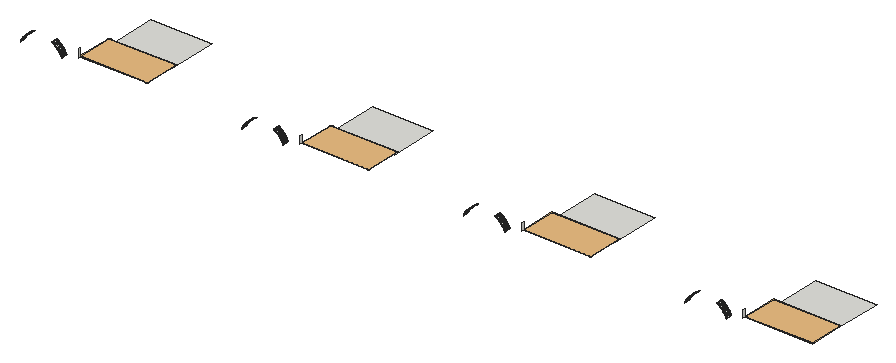
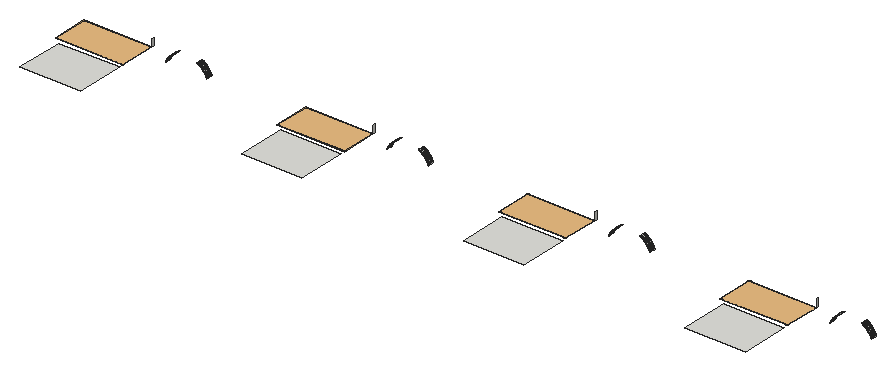
# SketchUp Ruby script. Lengths in inches.
U = 1.inch
M = Sketchup.active_model
def pt(a) = Geom::Point3d.new(a.map { |v| v * U })
def face(e, loops, mat)
  f = e.add_face(loops[0].map { |a| pt(a) })
  loops[1..].each { |l| e.add_face(l.map { |a| pt(a) }).erase! }
  f.material = f.back_material = mat if mat
  f
end
# faces: each face lists its corners as indices into pts; further lists are holes
def faces(e, pts, list, mat = nil) = list.each { |f| face(e, (f[0].is_a?(Array) ? f : [f]).map { |l| l.map { |i| pts[i] } }, mat) }
# xy, xz, yz: faces in a plane at the given z, y or x. An outline is a flat list of corners, or four numbers for a rectangle; further outlines are holes
def ring(l) = l.size == 4 ? [[l[0], l[1]], [l[2], l[1]], [l[2], l[3]], [l[0], l[3]]] : l.each_slice(2).to_a
def flat(e, list, mat, &to3) = list.each { |f| face(e, (f[0].is_a?(Array) ? f : [f]).map { |l| ring(l).map { |u, v| to3.(u, v) } }, mat) }
def xy(e, z, list, mat = nil) = flat(e, list, mat) { |x, y| [x, y, z] }
def xz(e, y, list, mat = nil) = flat(e, list, mat) { |x, z| [x, y, z] }
def yz(e, x, list, mat = nil) = flat(e, list, mat) { |y, z| [x, y, z] }
def lines(e, pts, list) = list.each { |a, b| e.add_line(pt(pts[a]), pt(pts[b])) }
# prism: a flat outline (further loops are holes) pulled along v
def prism(e, loops, v, mat = nil)
  f = face(e, loops, mat); d = Geom::Vector3d.new(v.map { |x| x * U })
  f.pushpull(f.normal.samedirection?(d) ? d.length : -d.length)
end
def box(e, o, s, mat = nil) = prism(e, [[o, [o[0] + s[0], o[1], o[2]], [o[0] + s[0], o[1] + s[1], o[2]], [o[0], o[1] + s[1], o[2]]]], [0, 0, s[2]], mat)
def at(x, y, z, deg = 0) = Geom::Transformation.translation(pt([x, y, z])) * Geom::Transformation.rotation(ORIGIN, Z_AXIS, deg.degrees)
def axes(o, x, y, z) = Geom::Transformation.new([*x, 0, *y, 0, *z, 0, *pt(o).to_a, 1])
def part(name) = M.definitions.add(name)
# library, detail: a bought-in or finely detailed component or shape, given as its bounding box
def library(name, o, s) = part(name).tap { |d| box(d.entities, o, s) }
def detail(e, o, s) = box(e.add_group.entities, o, s)
def put(e, d, t, mat = nil) = e.add_instance(d, t).tap { |i| i.material = mat if mat }
def group(e, t, mat = nil) = e.add_group.tap { |g| g.transformation = t; g.material = mat if mat }.entities
root = M.entities
M.materials.add("[Wood Cherry Original]").color = [152, 86, 42]
c1 = library("Group158\#2",[-67.5,-36,0],[135,72,0.25])
xy(root,249,[[301,301.25,422,398.125],[745,301.25,866,398.125],[1189,301.25,1310,398.125],[1633,301.25,1754,398.125]])
yz(root,294,[[224.6875,256,229.25,271]])
yz(root,738,[[224.6875,256,229.25,271]])
yz(root,1182,[[224.6875,256,229.25,271]])
yz(root,1626,[[224.6875,256,229.25,271]])
p = [[177.72,236.25,243.7],[177.72,224.6875,243.7],[177.48,224.6875,243.13],[177.48,236.25,243.13],[260.65,236.25,243.06],[260.65,224.6875,243.06],
  [260.41,224.6875,243.62],[260.41,236.25,243.62],[621.72,236.25,243.7],[621.72,224.6875,243.7],[621.48,224.6875,243.13],[621.48,236.25,243.13],
  [704.65,236.25,243.06],[704.65,224.6875,243.06],[704.41,224.6875,243.62],[704.41,236.25,243.62],[1065.72,236.25,243.7],[1065.72,224.6875,243.7],
  [1065.48,224.6875,243.13],[1065.48,236.25,243.13],[1148.65,236.25,243.06],[1148.65,224.6875,243.06],[1148.41,224.6875,243.62],[1148.41,236.25,243.62],
  [1509.72,236.25,243.7],[1509.72,224.6875,243.7],[1509.48,224.6875,243.13],[1509.48,236.25,243.13],[1592.65,236.25,243.06],[1592.65,224.6875,243.06],
  [1592.41,224.6875,243.62],[1592.41,236.25,243.62],[260.17,224.6875,244.18],[260.17,236.25,244.18],[704.17,224.6875,244.18],[704.17,236.25,244.18],
  [1148.17,224.6875,244.18],[1148.17,236.25,244.18],[1592.17,224.6875,244.18],[1592.17,236.25,244.18],[177.97,236.25,244.26],[177.97,224.6875,244.26],
  [621.97,236.25,244.26],[621.97,224.6875,244.26],[1065.97,236.25,244.26],[1065.97,224.6875,244.26],[1509.97,236.25,244.26],[1509.97,224.6875,244.26],
  [259.92,224.6875,244.74],[259.92,236.25,244.74],[703.92,224.6875,244.74],[703.92,236.25,244.74],[1147.92,224.6875,244.74],[1147.92,236.25,244.74],
  [1591.92,224.6875,244.74],[1591.92,236.25,244.74],[178.22,236.25,244.83],[178.22,224.6875,244.83],[622.22,236.25,244.83],[622.22,224.6875,244.83],
  [1066.22,236.25,244.83],[1066.22,224.6875,244.83],[1510.22,236.25,244.83],[1510.22,224.6875,244.83],[259.66,224.6875,245.3],[259.66,236.25,245.3],
  [703.66,224.6875,245.3],[703.66,236.25,245.3],[1147.66,224.6875,245.3],[1147.66,236.25,245.3],[1591.66,224.6875,245.3],[1591.66,236.25,245.3],
  [178.48,236.25,245.38],[178.48,224.6875,245.38],[622.48,236.25,245.38],[622.48,224.6875,245.38],[1066.48,236.25,245.38],[1066.48,224.6875,245.38],
  [1510.48,236.25,245.38],[1510.48,224.6875,245.38],[259.39,224.6875,245.85],[259.39,236.25,245.85],[703.39,224.6875,245.85],[703.39,236.25,245.85],
  [1147.39,224.6875,245.85],[1147.39,236.25,245.85],[1591.39,224.6875,245.85],[1591.39,236.25,245.85],[178.75,236.25,245.94],[178.75,224.6875,245.94],
  [622.75,236.25,245.94],[622.75,224.6875,245.94],[1066.75,236.25,245.94],[1066.75,224.6875,245.94],[1510.75,236.25,245.94],[1510.75,224.6875,245.94],
  [259.12,224.6875,246.39],[259.12,236.25,246.39],[703.12,224.6875,246.39],[703.12,236.25,246.39],[1147.12,224.6875,246.39],[1147.12,236.25,246.39],
  [1591.12,224.6875,246.39],[1591.12,236.25,246.39],[179.02,236.25,246.49],[179.02,224.6875,246.49],[623.02,236.25,246.49],[623.02,224.6875,246.49],
  [1067.02,236.25,246.49],[1067.02,224.6875,246.49],[1511.02,236.25,246.49],[1511.02,224.6875,246.49],[258.84,224.6875,246.9375],[258.84,236.25,246.9375],
  [702.84,224.6875,246.9375],[702.84,236.25,246.9375],[1146.84,224.6875,246.9375],[1146.84,236.25,246.9375],[1590.84,224.6875,246.9375],[1590.84,236.25,246.9375],
  [179.31,236.25,247.04],[179.31,224.6875,247.04],[623.31,236.25,247.04],[623.31,224.6875,247.04],[1067.31,236.25,247.04],[1067.31,224.6875,247.04],
  [1511.31,236.25,247.04],[1511.31,224.6875,247.04],[258.55,224.6875,247.48],[258.55,236.25,247.48],[702.55,224.6875,247.48],[702.55,236.25,247.48],
  [1146.55,224.6875,247.48],[1146.55,236.25,247.48],[1590.55,224.6875,247.48],[1590.55,236.25,247.48],[179.6,236.25,247.58],[179.6,224.6875,247.58],
  [623.6,236.25,247.58],[623.6,224.6875,247.58],[1067.6,236.25,247.58],[1067.6,224.6875,247.58],[1511.6,236.25,247.58],[1511.6,224.6875,247.58],
  [258.26,224.6875,248.01],[258.26,236.25,248.01],[702.26,224.6875,248.01],[702.26,236.25,248.01],[1146.26,224.6875,248.01],[1146.26,236.25,248.01],
  [1590.26,224.6875,248.01],[1590.26,236.25,248.01],[179.9,236.25,248.12],[179.9,224.6875,248.12],[623.9,236.25,248.12],[623.9,224.6875,248.12],
  [1067.9,236.25,248.12],[1067.9,224.6875,248.12],[1511.9,236.25,248.12],[1511.9,224.6875,248.12],[257.95,224.6875,248.54],[257.95,236.25,248.54],
  [701.95,224.6875,248.54],[701.95,236.25,248.54],[1145.95,224.6875,248.54],[1145.95,236.25,248.54],[1589.95,224.6875,248.54],[1589.95,236.25,248.54],
  [180.2,236.25,248.66],[180.2,224.6875,248.66],[624.2,236.25,248.66],[624.2,224.6875,248.66],[1068.2,236.25,248.66],[1068.2,224.6875,248.66],
  [1512.2,236.25,248.66],[1512.2,224.6875,248.66],[257.64,224.6875,249.07],[257.64,236.25,249.07],[701.64,224.6875,249.07],[701.64,236.25,249.07],
  [1145.64,224.6875,249.07],[1145.64,236.25,249.07],[1589.64,224.6875,249.07],[1589.64,236.25,249.07],[180.52,236.25,249.19],[180.52,224.6875,249.19],
  [624.52,236.25,249.19],[624.52,224.6875,249.19],[1068.52,236.25,249.19],[1068.52,224.6875,249.19],[1512.52,236.25,249.19],[1512.52,224.6875,249.19],
  [257.33,224.6875,249.59],[257.33,236.25,249.59],[701.33,224.6875,249.59],[701.33,236.25,249.59],[1145.33,224.6875,249.59],[1145.33,236.25,249.59],
  [1589.33,224.6875,249.59],[1589.33,236.25,249.59],[180.84,236.25,249.72],[180.84,224.6875,249.72],[624.84,236.25,249.72],[624.84,224.6875,249.72],
  [1068.84,236.25,249.72],[1068.84,224.6875,249.72],[1512.84,236.25,249.72],[1512.84,224.6875,249.72],[257,224.6875,250.11],[257,236.25,250.11],
  [701,224.6875,250.11],[701,236.25,250.11],[1145,224.6875,250.11],[1145,236.25,250.11],[1589,224.6875,250.11],[1589,236.25,250.11],
  [181.16,236.25,250.24],[181.16,224.6875,250.24],[625.16,236.25,250.24],[625.16,224.6875,250.24],[1069.16,236.25,250.24],[1069.16,224.6875,250.24],
  [1513.16,236.25,250.24],[1513.16,224.6875,250.24],[256.67,224.6875,250.625],[256.67,236.25,250.625],[700.67,224.6875,250.625],[700.67,236.25,250.625],
  [1144.67,224.6875,250.625],[1144.67,236.25,250.625],[1588.67,224.6875,250.625],[1588.67,236.25,250.625],[181.5,236.25,250.76],[181.5,224.6875,250.76],
  [625.5,236.25,250.76],[625.5,224.6875,250.76],[1069.5,236.25,250.76],[1069.5,224.6875,250.76],[1513.5,236.25,250.76],[1513.5,224.6875,250.76],
  [256.33,224.6875,251.13],[256.33,236.25,251.13],[700.33,224.6875,251.13],[700.33,236.25,251.13],[1144.33,224.6875,251.13],[1144.33,236.25,251.13],
  [1588.33,224.6875,251.13],[1588.33,236.25,251.13],[181.84,236.25,251.27],[181.84,224.6875,251.27],[625.84,236.25,251.27],[625.84,224.6875,251.27],
  [1069.84,236.25,251.27],[1069.84,224.6875,251.27],[1513.84,236.25,251.27],[1513.84,224.6875,251.27],[255.99,224.6875,251.64],[255.99,236.25,251.64],
  [699.99,224.6875,251.64],[699.99,236.25,251.64],[1143.99,224.6875,251.64],[1143.99,236.25,251.64],[1587.99,224.6875,251.64],[1587.99,236.25,251.64],
  [182.19,236.25,251.78],[182.19,224.6875,251.78],[626.19,236.25,251.78],[626.19,224.6875,251.78],[1070.19,236.25,251.78],[1070.19,224.6875,251.78],
  [1514.19,236.25,251.78],[1514.19,224.6875,251.78],[255.64,224.6875,252.14],[255.64,236.25,252.14],[699.64,224.6875,252.14],[699.64,236.25,252.14],
  [1143.64,224.6875,252.14],[1143.64,236.25,252.14],[1587.64,224.6875,252.14],[1587.64,236.25,252.14],[182.55,236.25,252.28],[182.55,224.6875,252.28],
  [626.55,236.25,252.28],[626.55,224.6875,252.28],[1070.55,236.25,252.28],[1070.55,224.6875,252.28],[1514.55,236.25,252.28],[1514.55,224.6875,252.28],
  [255.28,224.6875,252.63],[255.28,236.25,252.63],[699.28,224.6875,252.63],[699.28,236.25,252.63],[1143.28,224.6875,252.63],[1143.28,236.25,252.63],
  [1587.28,224.6875,252.63],[1587.28,236.25,252.63],[182.91,236.25,252.78],[182.91,224.6875,252.78],[626.91,236.25,252.78],[626.91,224.6875,252.78],
  [1070.91,236.25,252.78],[1070.91,224.6875,252.78],[1514.91,236.25,252.78],[1514.91,224.6875,252.78],[254.91,224.6875,253.125],[254.91,236.25,253.125],
  [698.91,224.6875,253.125],[698.91,236.25,253.125],[1142.91,224.6875,253.125],[1142.91,236.25,253.125],[1586.91,224.6875,253.125],[1586.91,236.25,253.125],
  [183.28,236.25,253.27],[183.28,224.6875,253.27],[627.28,236.25,253.27],[627.28,224.6875,253.27],[1071.28,236.25,253.27],[1071.28,224.6875,253.27],
  [1515.28,236.25,253.27],[1515.28,224.6875,253.27],[254.54,224.6875,253.61],[254.54,236.25,253.61],[698.54,224.6875,253.61],[698.54,236.25,253.61],
  [1142.54,224.6875,253.61],[1142.54,236.25,253.61],[1586.54,224.6875,253.61],[1586.54,236.25,253.61],[183.65,236.25,253.76],[183.65,224.6875,253.76],
  [627.65,236.25,253.76],[627.65,224.6875,253.76],[1071.65,236.25,253.76],[1071.65,224.6875,253.76],[1515.65,236.25,253.76],[1515.65,224.6875,253.76],
  [254.16,224.6875,254.09],[254.16,236.25,254.09],[698.16,224.6875,254.09],[698.16,236.25,254.09],[1142.16,224.6875,254.09],[1142.16,236.25,254.09],
  [1586.16,224.6875,254.09],[1586.16,236.25,254.09],[184.04,236.25,254.25],[184.04,224.6875,254.25],[628.04,236.25,254.25],[628.04,224.6875,254.25],
  [1072.04,236.25,254.25],[1072.04,224.6875,254.25],[1516.04,236.25,254.25],[1516.04,224.6875,254.25],[253.78,224.6875,254.5625],[253.78,236.25,254.5625],
  [697.78,224.6875,254.5625],[697.78,236.25,254.5625],[1141.78,224.6875,254.5625],[1141.78,236.25,254.5625],[1585.78,224.6875,254.5625],[1585.78,236.25,254.5625],
  [184.43,236.25,254.72],[184.43,224.6875,254.72],[628.43,236.25,254.72],[628.43,224.6875,254.72],[1072.43,236.25,254.72],[1072.43,224.6875,254.72],
  [1516.43,236.25,254.72],[1516.43,224.6875,254.72],[253.39,224.6875,255.03],[253.39,236.25,255.03],[697.39,224.6875,255.03],[697.39,236.25,255.03],
  [1141.39,224.6875,255.03],[1141.39,236.25,255.03],[1585.39,224.6875,255.03],[1585.39,236.25,255.03],[184.82,236.25,255.2],[184.82,224.6875,255.2],
  [628.82,236.25,255.2],[628.82,224.6875,255.2],[1072.82,236.25,255.2],[1072.82,224.6875,255.2],[1516.82,236.25,255.2],[1516.82,224.6875,255.2],
  [252.99,224.6875,255.5],[252.99,236.25,255.5],[696.99,224.6875,255.5],[696.99,236.25,255.5],[1140.99,224.6875,255.5],[1140.99,236.25,255.5],
  [1584.99,224.6875,255.5],[1584.99,236.25,255.5],[185.23,236.25,255.66],[185.23,224.6875,255.66],[629.23,236.25,255.66],[629.23,224.6875,255.66],
  [1073.23,236.25,255.66],[1073.23,224.6875,255.66],[1517.23,236.25,255.66],[1517.23,224.6875,255.66],[252.58,224.6875,255.96],[252.58,236.25,255.96],
  [696.58,224.6875,255.96],[696.58,236.25,255.96],[1140.58,224.6875,255.96],[1140.58,236.25,255.96],[1584.58,224.6875,255.96],[1584.58,236.25,255.96],
  [185.64,236.25,256.125],[185.64,224.6875,256.125],[629.64,236.25,256.125],[629.64,224.6875,256.125],[1073.64,236.25,256.125],[1073.64,224.6875,256.125],
  [1517.64,236.25,256.125],[1517.64,224.6875,256.125],[252.17,224.6875,256.41],[252.17,236.25,256.41],[696.17,224.6875,256.41],[696.17,236.25,256.41],
  [1140.17,224.6875,256.41],[1140.17,236.25,256.41],[1584.17,224.6875,256.41],[1584.17,236.25,256.41],[186.05,236.25,256.58],[186.05,224.6875,256.58],
  [630.05,236.25,256.58],[630.05,224.6875,256.58],[1074.05,236.25,256.58],[1074.05,224.6875,256.58],[1518.05,236.25,256.58],[1518.05,224.6875,256.58],
  [251.76,224.6875,256.86],[251.76,236.25,256.86],[695.76,224.6875,256.86],[695.76,236.25,256.86],[1139.76,224.6875,256.86],[1139.76,236.25,256.86],
  [1583.76,224.6875,256.86],[1583.76,236.25,256.86],[186.47,236.25,257.03],[186.47,224.6875,257.03],[630.47,236.25,257.03],[630.47,224.6875,257.03],
  [1074.47,236.25,257.03],[1074.47,224.6875,257.03],[1518.47,236.25,257.03],[1518.47,224.6875,257.03],[251.34,224.6875,257.3],[251.34,236.25,257.3],
  [695.34,224.6875,257.3],[695.34,236.25,257.3],[1139.34,224.6875,257.3],[1139.34,236.25,257.3],[1583.34,224.6875,257.3],[1583.34,236.25,257.3],
  [186.9,236.25,257.48],[186.9,224.6875,257.48],[630.9,236.25,257.48],[630.9,224.6875,257.48],[1074.9,236.25,257.48],[1074.9,224.6875,257.48],
  [1518.9,236.25,257.48],[1518.9,224.6875,257.48],[250.91,224.6875,257.74],[250.91,236.25,257.74],[694.91,224.6875,257.74],[694.91,236.25,257.74],
  [1138.91,224.6875,257.74],[1138.91,236.25,257.74],[1582.91,224.6875,257.74],[1582.91,236.25,257.74],[187.33,236.25,257.91],[187.33,224.6875,257.91],
  [631.33,236.25,257.91],[631.33,224.6875,257.91],[1075.33,236.25,257.91],[1075.33,224.6875,257.91],[1519.33,236.25,257.91],[1519.33,224.6875,257.91],
  [250.47,224.6875,258.17],[250.47,236.25,258.17],[694.47,224.6875,258.17],[694.47,236.25,258.17],[1138.47,224.6875,258.17],[1138.47,236.25,258.17],
  [1582.47,224.6875,258.17],[1582.47,236.25,258.17],[187.77,236.25,258.35],[187.77,224.6875,258.35],[631.77,236.25,258.35],[631.77,224.6875,258.35],
  [1075.77,236.25,258.35],[1075.77,224.6875,258.35],[1519.77,236.25,258.35],[1519.77,224.6875,258.35],[250.03,224.6875,258.59],[250.03,236.25,258.59],
  [694.03,224.6875,258.59],[694.03,236.25,258.59],[1138.03,224.6875,258.59],[1138.03,236.25,258.59],[1582.03,224.6875,258.59],[1582.03,236.25,258.59],
  [188.22,236.25,258.77],[188.22,224.6875,258.77],[632.22,236.25,258.77],[632.22,224.6875,258.77],[1076.22,236.25,258.77],[1076.22,224.6875,258.77],
  [1520.22,236.25,258.77],[1520.22,224.6875,258.77],[249.59,224.6875,259.01],[249.59,236.25,259.01],[693.59,224.6875,259.01],[693.59,236.25,259.01],
  [1137.59,224.6875,259.01],[1137.59,236.25,259.01],[1581.59,224.6875,259.01],[1581.59,236.25,259.01],[188.67,236.25,259.19],[188.67,224.6875,259.19],
  [632.67,236.25,259.19],[632.67,224.6875,259.19],[1076.67,236.25,259.19],[1076.67,224.6875,259.19],[1520.67,236.25,259.19],[1520.67,224.6875,259.19],
  [249.14,224.6875,259.42],[249.14,236.25,259.42],[693.14,224.6875,259.42],[693.14,236.25,259.42],[1137.14,224.6875,259.42],[1137.14,236.25,259.42],
  [1581.14,224.6875,259.42],[1581.14,236.25,259.42],[189.13,236.25,259.61],[189.13,224.6875,259.61],[633.13,236.25,259.61],[633.13,224.6875,259.61],
  [1077.13,236.25,259.61],[1077.13,224.6875,259.61],[1521.13,236.25,259.61],[1521.13,224.6875,259.61],[248.68,224.6875,259.83],[248.68,236.25,259.83],
  [692.68,224.6875,259.83],[692.68,236.25,259.83],[1136.68,224.6875,259.83],[1136.68,236.25,259.83],[1580.68,224.6875,259.83],[1580.68,236.25,259.83],
  [189.59,236.25,260.02],[189.59,224.6875,260.02],[633.59,236.25,260.02],[633.59,224.6875,260.02],[1077.59,236.25,260.02],[1077.59,224.6875,260.02],
  [1521.59,236.25,260.02],[1521.59,224.6875,260.02],[248.22,224.6875,260.23],[248.22,236.25,260.23],[692.22,224.6875,260.23],[692.22,236.25,260.23],
  [1136.22,224.6875,260.23],[1136.22,236.25,260.23],[1580.22,224.6875,260.23],[1580.22,236.25,260.23],[190.06,236.25,260.42],[190.06,224.6875,260.42],
  [634.06,236.25,260.42],[634.06,224.6875,260.42],[1078.06,236.25,260.42],[1078.06,224.6875,260.42],[1522.06,236.25,260.42],[1522.06,224.6875,260.42],
  [247.75,224.6875,260.625],[247.75,236.25,260.625],[691.75,224.6875,260.625],[691.75,236.25,260.625],[1135.75,224.6875,260.625],[1135.75,236.25,260.625],
  [1579.75,224.6875,260.625],[1579.75,236.25,260.625],[190.53,236.25,260.8125],[190.53,224.6875,260.8125],[634.53,236.25,260.8125],[634.53,224.6875,260.8125],
  [1078.53,236.25,260.8125],[1078.53,224.6875,260.8125],[1522.53,236.25,260.8125],[1522.53,224.6875,260.8125],[247.28,224.6875,261.01],[247.28,236.25,261.01],
  [691.28,224.6875,261.01],[691.28,236.25,261.01],[1135.28,224.6875,261.01],[1135.28,236.25,261.01],[1579.28,224.6875,261.01],[1579.28,236.25,261.01],
  [191.01,236.25,261.2],[191.01,224.6875,261.2],[635.01,236.25,261.2],[635.01,224.6875,261.2],[1079.01,236.25,261.2],[1079.01,224.6875,261.2],
  [1523.01,236.25,261.2],[1523.01,224.6875,261.2],[246.8,224.6875,261.39],[246.8,236.25,261.39],[690.8,224.6875,261.39],[690.8,236.25,261.39],
  [1134.8,224.6875,261.39],[1134.8,236.25,261.39],[1578.8,224.6875,261.39],[1578.8,236.25,261.39],[191.5,236.25,261.58],[191.5,224.6875,261.58],
  [635.5,236.25,261.58],[635.5,224.6875,261.58],[1079.5,236.25,261.58],[1079.5,224.6875,261.58],[1523.5,236.25,261.58],[1523.5,224.6875,261.58],
  [246.3125,224.6875,261.77],[246.3125,236.25,261.77],[690.3125,224.6875,261.77],[690.3125,236.25,261.77],[1134.3125,224.6875,261.77],[1134.3125,236.25,261.77],
  [1578.3125,224.6875,261.77],[1578.3125,236.25,261.77],[191.99,236.25,261.96],[191.99,224.6875,261.96],[635.99,236.25,261.96],[635.99,224.6875,261.96],
  [1079.99,236.25,261.96],[1079.99,224.6875,261.96],[1523.99,236.25,261.96],[1523.99,224.6875,261.96],[245.82,224.6875,262.13],[245.82,236.25,262.13],
  [689.82,224.6875,262.13],[689.82,236.25,262.13],[1133.82,224.6875,262.13],[1133.82,236.25,262.13],[1577.82,224.6875,262.13],[1577.82,236.25,262.13],
  [192.48,236.25,262.32],[192.48,224.6875,262.32],[636.48,236.25,262.32],[636.48,224.6875,262.32],[1080.48,236.25,262.32],[1080.48,224.6875,262.32],
  [1524.48,236.25,262.32],[1524.48,224.6875,262.32],[245.33,224.6875,262.49],[245.33,236.25,262.49],[689.33,224.6875,262.49],[689.33,236.25,262.49],
  [1133.33,224.6875,262.49],[1133.33,236.25,262.49],[1577.33,224.6875,262.49],[1577.33,236.25,262.49],[192.98,236.25,262.68],[192.98,224.6875,262.68],
  [636.98,236.25,262.68],[636.98,224.6875,262.68],[1080.98,236.25,262.68],[1080.98,224.6875,262.68],[1524.98,236.25,262.68],[1524.98,224.6875,262.68],
  [244.83,224.6875,262.85],[244.83,236.25,262.85],[688.83,224.6875,262.85],[688.83,236.25,262.85],[1132.83,224.6875,262.85],[1132.83,236.25,262.85],
  [1576.83,224.6875,262.85],[1576.83,236.25,262.85],[193.49,236.25,263.04],[193.49,224.6875,263.04],[637.49,236.25,263.04],[637.49,224.6875,263.04],
  [1081.49,236.25,263.04],[1081.49,224.6875,263.04],[1525.49,236.25,263.04],[1525.49,224.6875,263.04],[244.33,224.6875,263.2],[244.33,236.25,263.2],
  [688.33,224.6875,263.2],[688.33,236.25,263.2],[1132.33,224.6875,263.2],[1132.33,236.25,263.2],[1576.33,224.6875,263.2],[1576.33,236.25,263.2],
  [194,236.25,263.39],[194,224.6875,263.39],[638,236.25,263.39],[638,224.6875,263.39],[1082,236.25,263.39],[1082,224.6875,263.39],
  [1526,236.25,263.39],[1526,224.6875,263.39],[243.82,224.6875,263.54],[243.82,236.25,263.54],[687.82,224.6875,263.54],[687.82,236.25,263.54],
  [1131.82,224.6875,263.54],[1131.82,236.25,263.54],[1575.82,224.6875,263.54],[1575.82,236.25,263.54],[194.51,236.25,263.73],[194.51,224.6875,263.73],
  [638.51,236.25,263.73],[638.51,224.6875,263.73],[1082.51,236.25,263.73],[1082.51,224.6875,263.73],[1526.51,236.25,263.73],[1526.51,224.6875,263.73],
  [243.31,224.6875,263.87],[243.31,236.25,263.87],[687.31,224.6875,263.87],[687.31,236.25,263.87],[1131.31,224.6875,263.87],[1131.31,236.25,263.87],
  [1575.31,224.6875,263.87],[1575.31,236.25,263.87],[195.03,236.25,264.06],[195.03,224.6875,264.06],[639.03,236.25,264.06],[639.03,224.6875,264.06],
  [1083.03,236.25,264.06],[1083.03,224.6875,264.06],[1527.03,236.25,264.06],[1527.03,224.6875,264.06],[242.79,224.6875,264.2],[242.79,236.25,264.2],
  [686.79,224.6875,264.2],[686.79,236.25,264.2],[1130.79,224.6875,264.2],[1130.79,236.25,264.2],[1574.79,224.6875,264.2],[1574.79,236.25,264.2],
  [195.55,236.25,264.39],[195.55,224.6875,264.39],[639.55,236.25,264.39],[639.55,224.6875,264.39],[1083.55,236.25,264.39],[1083.55,224.6875,264.39],
  [1527.55,236.25,264.39],[1527.55,224.6875,264.39],[242.27,224.6875,264.52],[242.27,236.25,264.52],[686.27,224.6875,264.52],[686.27,236.25,264.52],
  [1130.27,224.6875,264.52],[1130.27,236.25,264.52],[1574.27,224.6875,264.52],[1574.27,236.25,264.52],[196.08,236.25,264.7],[196.08,224.6875,264.7],
  [640.08,236.25,264.7],[640.08,224.6875,264.7],[1084.08,236.25,264.7],[1084.08,224.6875,264.7],[1528.08,236.25,264.7],[1528.08,224.6875,264.7],
  [241.75,224.6875,264.83],[241.75,236.25,264.83],[685.75,224.6875,264.83],[685.75,236.25,264.83],[1129.75,224.6875,264.83],[1129.75,236.25,264.83],
  [1573.75,224.6875,264.83],[1573.75,236.25,264.83],[196.61,236.25,265.02],[196.61,224.6875,265.02],[640.61,236.25,265.02],[640.61,224.6875,265.02],
  [1084.61,236.25,265.02],[1084.61,224.6875,265.02],[1528.61,236.25,265.02],[1528.61,224.6875,265.02],[241.22,224.6875,265.14],[241.22,236.25,265.14],
  [685.22,224.6875,265.14],[685.22,236.25,265.14],[1129.22,224.6875,265.14],[1129.22,236.25,265.14],[1573.22,224.6875,265.14],[1573.22,236.25,265.14],
  [197.15,236.25,265.32],[197.15,224.6875,265.32],[641.15,236.25,265.32],[641.15,224.6875,265.32],[1085.15,236.25,265.32],[1085.15,224.6875,265.32],
  [1529.15,236.25,265.32],[1529.15,224.6875,265.32]]
faces(root,p,[[0,1,2,3],[4,5,6,7],[8,9,10,11],[12,13,14,15],[16,17,18,19],[20,21,22,23],[24,25,26,27],[28,29,30,31],
  [7,6,32,33],[15,14,34,35],[23,22,36,37],[31,30,38,39],[40,41,1,0],[42,43,9,8],[44,45,17,16],[46,47,25,24],
  [33,32,48,49],[35,34,50,51],[37,36,52,53],[39,38,54,55],[56,57,41,40],[58,59,43,42],[60,61,45,44],[62,63,47,46],
  [49,48,64,65],[51,50,66,67],[53,52,68,69],[55,54,70,71],[72,73,57,56],[74,75,59,58],[76,77,61,60],[78,79,63,62],
  [65,64,80,81],[67,66,82,83],[69,68,84,85],[71,70,86,87],[88,89,73,72],[90,91,75,74],[92,93,77,76],[94,95,79,78],
  [81,80,96,97],[83,82,98,99],[85,84,100,101],[87,86,102,103],[104,105,89,88],[106,107,91,90],[108,109,93,92],[110,111,95,94],
  [97,96,112,113],[99,98,114,115],[101,100,116,117],[103,102,118,119],[120,121,105,104],[122,123,107,106],[124,125,109,108],[126,127,111,110],
  [113,112,128,129],[115,114,130,131],[117,116,132,133],[119,118,134,135],[136,137,121,120],[138,139,123,122],[140,141,125,124],[142,143,127,126],
  [129,128,144,145],[131,130,146,147],[133,132,148,149],[135,134,150,151],[152,153,137,136],[154,155,139,138],[156,157,141,140],[158,159,143,142],
  [145,144,160,161],[147,146,162,163],[149,148,164,165],[151,150,166,167],[168,169,153,152],[170,171,155,154],[172,173,157,156],[174,175,159,158],
  [161,160,176,177],[163,162,178,179],[165,164,180,181],[167,166,182,183],[184,185,169,168],[186,187,171,170],[188,189,173,172],[190,191,175,174],
  [177,176,192,193],[179,178,194,195],[181,180,196,197],[183,182,198,199],[200,201,185,184],[202,203,187,186],[204,205,189,188],[206,207,191,190],
  [193,192,208,209],[195,194,210,211],[197,196,212,213],[199,198,214,215],[216,217,201,200],[218,219,203,202],[220,221,205,204],[222,223,207,206],
  [209,208,224,225],[211,210,226,227],[213,212,228,229],[215,214,230,231],[232,233,217,216],[234,235,219,218],[236,237,221,220],[238,239,223,222],
  [225,224,240,241],[227,226,242,243],[229,228,244,245],[231,230,246,247],[248,249,233,232],[250,251,235,234],[252,253,237,236],[254,255,239,238],
  [241,240,256,257],[243,242,258,259],[245,244,260,261],[247,246,262,263],[264,265,249,248],[266,267,251,250],[268,269,253,252],[270,271,255,254],
  [257,256,272,273],[259,258,274,275],[261,260,276,277],[263,262,278,279],[280,281,265,264],[282,283,267,266],[284,285,269,268],[286,287,271,270],
  [273,272,288,289],[275,274,290,291],[277,276,292,293],[279,278,294,295],[296,297,281,280],[298,299,283,282],[300,301,285,284],[302,303,287,286],
  [289,288,304,305],[291,290,306,307],[293,292,308,309],[295,294,310,311],[312,313,297,296],[314,315,299,298],[316,317,301,300],[318,319,303,302],
  [305,304,320,321],[307,306,322,323],[309,308,324,325],[311,310,326,327],[328,329,313,312],[330,331,315,314],[332,333,317,316],[334,335,319,318],
  [321,320,336,337],[323,322,338,339],[325,324,340,341],[327,326,342,343],[344,345,329,328],[346,347,331,330],[348,349,333,332],[350,351,335,334],
  [337,336,352,353],[339,338,354,355],[341,340,356,357],[343,342,358,359],[360,361,345,344],[362,363,347,346],[364,365,349,348],[366,367,351,350],
  [353,352,368,369],[355,354,370,371],[357,356,372,373],[359,358,374,375],[376,377,361,360],[378,379,363,362],[380,381,365,364],[382,383,367,366],
  [369,368,384,385],[371,370,386,387],[373,372,388,389],[375,374,390,391],[392,393,377,376],[394,395,379,378],[396,397,381,380],[398,399,383,382],
  [385,384,400,401],[387,386,402,403],[389,388,404,405],[391,390,406,407],[408,409,393,392],[410,411,395,394],[412,413,397,396],[414,415,399,398],
  [401,400,416,417],[403,402,418,419],[405,404,420,421],[407,406,422,423],[424,425,409,408],[426,427,411,410],[428,429,413,412],[430,431,415,414],
  [417,416,432,433],[419,418,434,435],[421,420,436,437],[423,422,438,439],[440,441,425,424],[442,443,427,426],[444,445,429,428],[446,447,431,430],
  [433,432,448,449],[435,434,450,451],[437,436,452,453],[439,438,454,455],[456,457,441,440],[458,459,443,442],[460,461,445,444],[462,463,447,446],
  [449,448,464,465],[451,450,466,467],[453,452,468,469],[455,454,470,471],[472,473,457,456],[474,475,459,458],[476,477,461,460],[478,479,463,462],
  [465,464,480,481],[467,466,482,483],[469,468,484,485],[471,470,486,487],[488,489,473,472],[490,491,475,474],[492,493,477,476],[494,495,479,478],
  [481,480,496,497],[483,482,498,499],[485,484,500,501],[487,486,502,503],[504,505,489,488],[506,507,491,490],[508,509,493,492],[510,511,495,494],
  [497,496,512,513],[499,498,514,515],[501,500,516,517],[503,502,518,519],[520,521,505,504],[522,523,507,506],[524,525,509,508],[526,527,511,510],
  [513,512,528,529],[515,514,530,531],[517,516,532,533],[519,518,534,535],[536,537,521,520],[538,539,523,522],[540,541,525,524],[542,543,527,526],
  [529,528,544,545],[531,530,546,547],[533,532,548,549],[535,534,550,551],[552,553,537,536],[554,555,539,538],[556,557,541,540],[558,559,543,542],
  [545,544,560,561],[547,546,562,563],[549,548,564,565],[551,550,566,567],[568,569,553,552],[570,571,555,554],[572,573,557,556],[574,575,559,558],
  [561,560,576,577],[563,562,578,579],[565,564,580,581],[567,566,582,583],[584,585,569,568],[586,587,571,570],[588,589,573,572],[590,591,575,574],
  [577,576,592,593],[579,578,594,595],[581,580,596,597],[583,582,598,599],[600,601,585,584],[602,603,587,586],[604,605,589,588],[606,607,591,590],
  [593,592,608,609],[595,594,610,611],[597,596,612,613],[599,598,614,615],[616,617,601,600],[618,619,603,602],[620,621,605,604],[622,623,607,606],
  [609,608,624,625],[611,610,626,627],[613,612,628,629],[615,614,630,631],[632,633,617,616],[634,635,619,618],[636,637,621,620],[638,639,623,622],
  [625,624,640,641],[627,626,642,643],[629,628,644,645],[631,630,646,647],[648,649,633,632],[650,651,635,634],[652,653,637,636],[654,655,639,638],
  [641,640,656,657],[643,642,658,659],[645,644,660,661],[647,646,662,663],[664,665,649,648],[666,667,651,650],[668,669,653,652],[670,671,655,654],
  [657,656,672,673],[659,658,674,675],[661,660,676,677],[663,662,678,679],[680,681,665,664],[682,683,667,666],[684,685,669,668],[686,687,671,670],
  [673,672,688,689],[675,674,690,691],[677,676,692,693],[679,678,694,695],[696,697,681,680],[698,699,683,682],[700,701,685,684],[702,703,687,686],
  [689,688,704,705],[691,690,706,707],[693,692,708,709],[695,694,710,711],[712,713,697,696],[714,715,699,698],[716,717,701,700],[718,719,703,702],
  [705,704,720,721],[707,706,722,723],[709,708,724,725],[711,710,726,727],[728,729,713,712],[730,731,715,714],[732,733,717,716],[734,735,719,718],
  [721,720,736,737],[723,722,738,739],[725,724,740,741],[727,726,742,743],[744,745,729,728],[746,747,731,730],[748,749,733,732],[750,751,735,734],
  [737,736,752,753],[739,738,754,755],[741,740,756,757],[743,742,758,759],[760,761,745,744],[762,763,747,746],[764,765,749,748],[766,767,751,750],
  [753,752,768,769],[755,754,770,771],[757,756,772,773],[759,758,774,775],[776,777,761,760],[778,779,763,762],[780,781,765,764],[782,783,767,766],
  [769,768,784,785],[771,770,786,787],[773,772,788,789],[775,774,790,791],[792,793,777,776],[794,795,779,778],[796,797,781,780],[798,799,783,782]])
put(root,c1,at(361.5,265.25,256),"[Wood Cherry Original]")
put(root,c1,at(805.5,265.25,256),"[Wood Cherry Original]")
put(root,c1,at(1249.5,265.25,256),"[Wood Cherry Original]")
put(root,c1,at(1693.5,265.25,256),"[Wood Cherry Original]")
